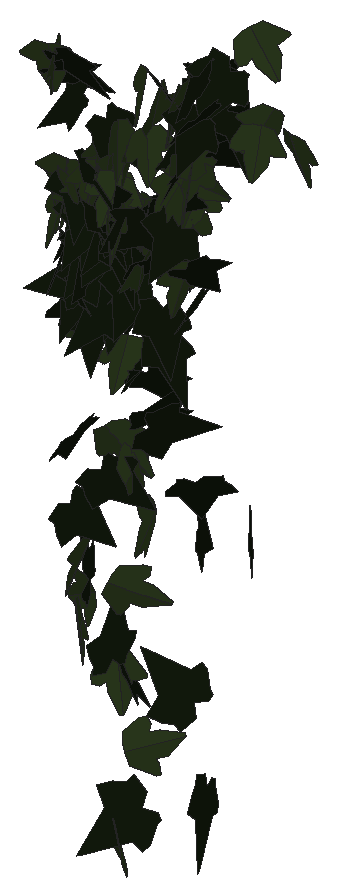
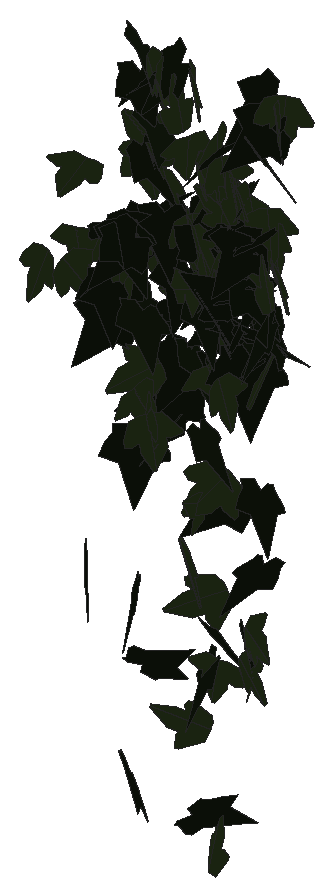
# SketchUp Ruby script. Lengths in inches.
U = 1.inch
M = Sketchup.active_model
def pt(a) = Geom::Point3d.new(a.map { |v| v * U })
def face(e, loops, mat)
  f = e.add_face(loops[0].map { |a| pt(a) })
  loops[1..].each { |l| e.add_face(l.map { |a| pt(a) }).erase! }
  f.material = f.back_material = mat if mat
  f
end
# faces: each face lists its corners as indices into pts; further lists are holes
def faces(e, pts, list, mat = nil) = list.each { |f| face(e, (f[0].is_a?(Array) ? f : [f]).map { |l| l.map { |i| pts[i] } }, mat) }
# xy, xz, yz: faces in a plane at the given z, y or x. An outline is a flat list of corners, or four numbers for a rectangle; further outlines are holes
def ring(l) = l.size == 4 ? [[l[0], l[1]], [l[2], l[1]], [l[2], l[3]], [l[0], l[3]]] : l.each_slice(2).to_a
def flat(e, list, mat, &to3) = list.each { |f| face(e, (f[0].is_a?(Array) ? f : [f]).map { |l| ring(l).map { |u, v| to3.(u, v) } }, mat) }
def xy(e, z, list, mat = nil) = flat(e, list, mat) { |x, y| [x, y, z] }
def xz(e, y, list, mat = nil) = flat(e, list, mat) { |x, z| [x, y, z] }
def yz(e, x, list, mat = nil) = flat(e, list, mat) { |y, z| [x, y, z] }
def lines(e, pts, list) = list.each { |a, b| e.add_line(pt(pts[a]), pt(pts[b])) }
# prism: a flat outline (further loops are holes) pulled along v
def prism(e, loops, v, mat = nil)
  f = face(e, loops, mat); d = Geom::Vector3d.new(v.map { |x| x * U })
  f.pushpull(f.normal.samedirection?(d) ? d.length : -d.length)
end
def box(e, o, s, mat = nil) = prism(e, [[o, [o[0] + s[0], o[1], o[2]], [o[0] + s[0], o[1] + s[1], o[2]], [o[0], o[1] + s[1], o[2]]]], [0, 0, s[2]], mat)
def at(x, y, z, deg = 0) = Geom::Transformation.translation(pt([x, y, z])) * Geom::Transformation.rotation(ORIGIN, Z_AXIS, deg.degrees)
def axes(o, x, y, z) = Geom::Transformation.new([*x, 0, *y, 0, *z, 0, *pt(o).to_a, 1])
def part(name) = M.definitions.add(name)
# library, detail: a bought-in or finely detailed component or shape, given as its bounding box
def library(name, o, s) = part(name).tap { |d| box(d.entities, o, s) }
def detail(e, o, s) = box(e.add_group.entities, o, s)
def put(e, d, t, mat = nil) = e.add_instance(d, t).tap { |i| i.material = mat if mat }
def group(e, t, mat = nil) = e.add_group.tap { |g| g.transformation = t; g.material = mat if mat }.entities
root = M.entities
M.materials.add("efeu1").color = [18, 25, 13]
M.materials.add("efeu2").color = [43, 57, 29]
c1 = part("ivyleaf_9")
p = [[1.54,2.16,1.25],[1.36,2.04,1.19],[-0.21,0.99,0.68],[-0.71,1.11,0.82],[-0.85,0.86,0.67],[-0.8,0.17,0.21],
  [-0.9,-0.01,0.1],[-0.67,-0.16,-0.02],[-0.08,-0.08,-0.05],[-0.03,-0.6,-0.4],[0.65,-0.88,-0.66],[0.83,-0.6,-0.49],
  [1.29,-0.42,-0.43],[1.8125,-0.07,-0.26],[1.21,0.44,0.15]]
faces(c1.entities,p,[[0,1,2,3,4,5,6,7,8,9,10,11,12,13,14]],"efeu1")
c2 = part("ivyleaf_10")
p = [[0,0.5,-0.03],[-0.0625,2.02,-0.43],[-0.19,2.01,-0.46],[-0.54,1.05,-0.29],[-0.52,0.625,-0.18],[-0.83,0.76,-0.28],
  [-1.16,0.64,-0.33],[-1.15,0.33,-0.24],[-0.77,-0.39,0.02],[-0.3,-0.51,0.16],[0.04,-0.48,0.23],[-0.02,2.01,-0.4375],
  [-0.06,2.01,-0.43],[0.04,-0.49,0.23],[0.67,-0.49,0.14],[1.38,0.36,-0.2],[1.375,0.51,-0.24],[0.81,0.65,-0.19],
  [0.62,0.59,-0.15],[0.6,1.09,-0.28],[0.5,1.23,-0.31]]
faces(c2.entities,p,[[0,1,2,3,4,5,6,7,8,9,10],[11,12,0,13,14,15,16,17,18,19,20]],"efeu2")
put(root,c1,axes([570.06,132.24,232.82],[0.80503,-0.25193,-0.4599],[-0.43444,0.15145,-0.84343],[0.29366,0.91468,0.01298]))
put(root,c2,axes([570.07,132.39,234.11],[0.35758,-0.85019,-0.25363],[0.0877,-0.23825,0.92226],[-0.88287,-0.36801,-0.01111]))
put(root,c1,axes([570.45,131.11,231.73],[0.17538,0.16443,1.06836],[0.09297,1.07602,-0.18087],[-1.07693,0.11967,0.15837]))
put(root,c2,axes([570.51,130.82,242.45],[-0.96058,-0.33509,0.03934],[-0.03215,-0.02726,-1.01724],[0.33585,-0.961,0.01514]))
put(root,c2,axes([570.41,131.36,234.92],[0.7141,-0.69206,-0.00415],[-0.00365,0.0022,-0.99443],[0.69207,0.71411,-0.00095]))
put(root,c2,axes([570.41,131.28,242.22],[0.48074,-0.88459,-0.03625],[0.07895,0.08391,-1.00083],[0.88181,0.47474,0.10937]))
put(root,c2,axes([570.74,131.15,236.51],[-0.90983,0.25476,0.26269],[-0.28872,-0.06724,-0.93478],[-0.22483,-0.9446,0.13739]))
put(root,c2,axes([571.03,132.55,216.36],[0.46106,-0.2348,-0.81317],[-0.63107,0.5217,-0.50845],[0.56402,0.77566,0.09583]))
put(root,c2,axes([570.85,139.36,230.89],[-0.69817,-0.66785,0.17498],[-0.06821,-0.18092,-0.96265],[0.68701,-0.69665,0.08225]))
put(root,c2,axes([570.59,132.8,218.12],[0.32909,-0.77667,0.49021],[0.17405,-0.45856,-0.84336],[0.90179,0.37193,-0.01612]))
put(root,c1,axes([571.32,132.36,217.23],[-0.49104,0.4243,-0.71417],[-0.76734,0.08611,0.57876],[0.31821,0.8624,0.29358]))
put(root,c2,axes([570.68,132.49,229.26],[-0.29802,0.71193,0.55488],[0.21221,-0.5127,0.77179],[0.87733,0.36585,0.0018]))
put(root,c1,axes([570.26,139.16,230.47],[0.36402,-0.90757,0.07302],[0.03277,-0.06553,-0.97783],[0.90991,0.36544,0.00601]))
put(root,c1,axes([571.44,131.79,231.68],[-0.80964,0.2299,0.44537],[-0.4632,-0.01997,-0.83173],[-0.19147,-0.92384,0.12881]))
put(root,c1,axes([571.05,131.61,224.2],[-0.16257,0.93149,-0.01676],[0.03186,-0.01144,-0.94512],[-0.9311,-0.16303,-0.02942]))
put(root,c2,axes([571.05,131.23,237.06],[-0.89178,-0.36298,0.18579],[-0.15683,-0.10711,-0.96202],[0.3764,-0.90461,0.03936]))
put(root,c1,axes([571.58,131.43,240.51],[-0.87516,0.48207,0.03648],[-0.03085,0.0196,-0.99914],[-0.48246,-0.8757,-0.00228]))
put(root,c1,axes([571.4,132,234.29],[-0.3315,0.76712,-0.46972],[0.06912,-0.47739,-0.82844],[-0.89684,-0.32034,0.10977]))
put(root,c1,axes([571.52,138.9,235.85],[-0.09953,0.94835,0.08723],[-0.17627,0.06785,-0.93873],[-0.9359,-0.11363,0.16752]))
put(root,c2,axes([570.63,139.5,231.6875],[0.54974,-0.43926,0.63584],[0.64486,-0.1693,-0.6745],[0.42591,0.82331,0.20054]))
put(root,c2,axes([571.24,133.97,230.12],[-0.02569,-0.94211,0.10099],[0.00022,-0.10103,-0.94246],[0.94751,-0.02552,0.00296]))
put(root,c1,axes([570.76,131.08,241.6],[0.86003,0.47043,0.25534],[0.19952,0.16666,-0.97907],[-0.49668,0.88152,0.04884]))
put(root,c1,axes([571.36,131.87,230.49],[0.4534,0.97062,-0.41574],[-0.18987,-0.37013,-1.0712],[-1.03869,0.49134,0.01433]))
put(root,c1,axes([570.94,131.71,220.78],[0.20367,-0.42553,-0.82993],[-0.16032,0.82087,-0.46023],[0.91878,0.23757,0.10367]))
put(root,c1,axes([571.66,134.79,228.26],[-0.57972,0.70231,-0.26845],[0.14614,-0.22727,-0.91015],[-0.73753,-0.59707,0.03067]))
put(root,c2,axes([571.375,139.47,232.26],[0.3097,0.78323,-0.43615],[-0.30156,-0.34354,-0.83104],[-0.84424,0.41003,0.13685]))
put(root,c2,axes([571.46,131.82,235.83],[-0.32952,-0.86435,0.28217],[-0.03389,-0.28825,-0.92253],[0.90861,-0.32421,0.06793]))
put(root,c1,axes([571.18,131.99,236.23],[-0.17021,-0.95833,0.01524],[0.01859,-0.01877,-0.97309],[0.95827,-0.16985,0.02159]))
put(root,c1,axes([571.5,131.72,231.66],[-0.80182,-0.36143,-0.36519],[0.3775,0.04477,-0.87315],[0.34855,-0.87993,0.10558]))
put(root,c1,axes([571.44,131.9,236.125],[0.53595,0.77957,0.25222],[0.14579,0.20585,-0.94602],[-0.80628,0.55541,-0.00339]))
put(root,c1,axes([571.24,130.55,242.59],[0.993,0.18995,0.03398],[0.03615,-0.00816,-1.0109],[-0.18955,0.99355,-0.0148]))
put(root,c1,axes([571.47,132.28,229.91],[-0.03325,-0.9598,-0.02296],[-0.01292,0.02342,-0.96028],[0.95999,-0.03293,-0.01372]))
put(root,c2,axes([571.39,131.58,215.92],[-0.33428,0.62383,-0.84867],[0.39543,-0.75093,-0.70773],[-0.97624,-0.51778,0.00393]))
put(root,c1,axes([571.3,131.54,231.25],[0.77282,-0.60709,0.0565],[0.04099,-0.03928,-0.98274],[0.60834,0.77389,-0.00556]))
put(root,c1,axes([572,131.83,235.03],[-0.74465,-0.60263,-0.04579],[0.04449,0.0178,-0.95784],[0.60272,-0.74585,0.01413]))
put(root,c2,axes([571.37,138.6875,233.17],[0.48259,0.11114,0.84976],[0.48705,0.76686,-0.37689],[-0.70515,0.60573,0.32124]))
put(root,c1,axes([572.02,132.18,233.34],[-0.57787,-0.7499,0.17358],[-0.10287,-0.13987,-0.94671],[0.76282,-0.58694,0.00383]))
put(root,c1,axes([571.59,132.27,232.28],[0.27664,-0.27868,-0.87738],[0.62504,-0.61575,0.39266],[-0.67587,-0.68351,0.004]))
put(root,c2,axes([572.3125,131.54,237.27],[-0.2833,-0.90798,0.17177],[0.0667,-0.19929,-0.94341],[0.92168,-0.26467,0.12107]))
put(root,c1,axes([572.08,132.1,236.54],[-0.47191,-0.66497,-0.52291],[0.30279,0.42633,-0.81541],[0.7899,-0.5607,0.00016]))
put(root,c2,axes([572.76,137.95,236.44],[-0.30967,0.6152,0.70883],[-0.49007,0.5306,-0.67461],[-0.80047,-0.56285,0.1388]))
put(root,c2,axes([572.45,131.34,237.875],[0.65649,-0.72856,0.031],[0.04525,-0.00094,-0.98015],[0.72782,0.65722,0.03297]))
put(root,c1,axes([572.91,138.375,238.94],[-0.16515,0.90966,-0.30338],[-0.0851,-0.32053,-0.91477],[-0.95513,-0.12873,0.13396]))
put(root,c2,axes([572.33,131.79,237.34],[0.37838,-0.88399,-0.20248],[0.06558,-0.19215,0.96145],[-0.90451,-0.38373,-0.015]))
put(root,c1,axes([572.16,132.23,233.17],[-0.12118,-0.04696,0.95522],[0.90753,0.29812,0.12979],[-0.30172,0.91556,0.00673]))
put(root,c1,axes([572.15,131.46,237.55],[0.57878,-0.79009,-0.00887],[0.00347,0.01353,-0.97934],[0.79013,0.57869,0.01079]))
put(root,c1,axes([572.36,138.53,238.96],[0.90513,0.36895,0.04233],[0.03833,0.01809,-0.97743],[-0.36939,0.90594,0.00228]))
put(root,c1,axes([572.26,131.79,235.17],[0.50367,-0.8208,-0.00799],[0.0468,0.03807,-0.96116],[0.81951,0.50229,0.0598]))
put(root,c2,axes([572.47,131.73,237.125],[-0.4335,-0.53228,0.70794],[0.44133,0.55357,0.68646],[-0.76795,0.6186,-0.00514]))
put(root,c1,axes([573.25,131.16,231.32],[-0.98427,-0.05458,-0.09049],[0.09,0.01136,-0.98577],[0.05538,-0.98836,-0.00633]))
put(root,c1,axes([573.1,138.91,236.83],[0.31007,0.86617,-0.28105],[-0.13665,-0.24928,-0.91901],[-0.90032,0.33614,0.04269]))
put(root,c2,axes([573.11,131.55,238.95],[-0.24491,-0.9614,-0.02234],[-0.00535,0.02441,-0.99204],[0.96164,-0.24471,-0.0112]))
put(root,c2,axes([573.17,138.45,238.46],[-0.72614,-0.64271,0.01976],[-0.01782,-0.00969,-0.96971],[0.64277,-0.72634,-0.00455]))
put(root,c1,axes([573.68,132.07,232.42],[-0.38396,0.56598,0.6905],[-0.39616,0.5656,-0.68389],[-0.80012,-0.55165,0.00726]))
put(root,c2,axes([572.71,132.32,224.52],[-0.92825,-0.10382,-0.68038],[0.6769,0.06889,-0.93403],[0.12447,-1.14883,0.00548]))
put(root,c1,axes([573.4,131.67,235.11],[-0.94364,-0.06464,-0.21251],[0.21457,-0.02559,-0.94503],[0.0574,-0.96693,0.03922]))
put(root,c2,axes([572.68,132.18,231.24],[0.6016,-0.3423,0.67466],[0.58303,-0.33951,-0.69215],[0.48209,0.83775,-0.00484]))
put(root,c1,axes([573.09,132.22,231.59],[-0.37575,-0.88439,-0.09622],[0.02409,0.0943,-0.96079],[0.88928,-0.37624,-0.01463]))
put(root,c2,axes([573.09,131.73,235.16],[-0.17439,0.78244,-0.53018],[0.10337,-0.52011,-0.80157],[-0.93948,-0.20247,0.01022]))
put(root,c1,axes([572.85,131.39,223.22],[-0.01193,-0.22479,-0.93849],[0.23992,0.90841,-0.22063],[0.93474,-0.23603,0.04465]))
put(root,c1,axes([573.11,138.71,235.2],[0.6846,0.68212,0.23219],[0.15541,0.17296,-0.96634],[-0.7036,0.70191,0.01248]))
put(root,c1,axes([573.75,132.04,232.42],[-0.24131,0.93783,0.0854],[-0.01278,0.08489,-0.96834],[-0.94162,-0.24149,-0.00875]))
put(root,c1,axes([572.96,132.11,233.6],[0.36008,-0.89443,0.10005],[0.04822,-0.08844,-0.96412],[0.89871,0.36311,0.01164]))
put(root,c2,axes([573.54,132,234.63],[0.09297,-0.93451,0.23239],[-0.0068,-0.2341,-0.93867],[0.96294,0.08857,-0.02907]))
put(root,c2,axes([573.47,131.34,236.97],[0.8917,0.3146,-0.20741],[-0.1995,-0.05787,-0.9455],[-0.31967,0.91367,0.01153]))
put(root,c2,axes([574.08,132.34,235.65],[-0.7996,-0.00173,0.54563],[-0.53066,-0.22275,-0.77836],[0.12694,-0.94205,0.18304]))
put(root,c2,axes([573.62,132.07,223.05],[0.0878,0.40548,-0.90284],[0.10019,0.89809,0.41309],[0.98464,-0.12754,0.03847]))
put(root,c1,axes([573.68,132.19,232.28],[-0.81495,-0.45221,-0.25531],[0.28306,0.01149,-0.92389],[0.43537,-0.85393,0.12277]))
put(root,c1,axes([573.16,131.3,239.88],[0.51193,-0.72194,-0.47513],[-0.03785,0.53297,-0.85061],[0.86343,0.4514,0.24442]))
put(root,c1,axes([573.75,138.42,239.21],[-0.60571,-0.75027,0.13069],[-0.1021,-0.08547,-0.96392],[0.7547,-0.61373,-0.02552]))
put(root,c2,axes([573.65,131.77,229.18],[0.48466,0.78049,-0.29783],[-0.16497,-0.24813,-0.91868],[-0.81893,0.51189,0.0088]))
put(root,c1,axes([574.08,130.41,215.36],[-0.92822,0.41046,-0.14762],[-0.14699,0.03244,1.0145],[0.41068,0.93933,0.02947]))
put(root,c1,axes([573.82,132.01,235.03],[0.51456,0.37373,0.736],[-0.58363,-0.44861,0.63582],[0.58374,-0.77796,-0.01307]))
put(root,c2,axes([573.67,131.13,235.86],[0.85576,-0.40605,0.19881],[0.19672,-0.04877,-0.94639],[0.40707,0.87719,0.03942]))
put(root,c2,axes([573.93,131.16,205.52],[-0.8462,0.58583,0.16938],[0.13526,-0.10219,1.02918],[0.59463,0.85692,0.00694]))
put(root,c1,axes([573.49,139.1875,236.92],[0.1829,-0.94512,-0.01882],[0.07328,0.03329,-0.95947],[0.94246,0.18083,0.07826]))
put(root,c2,axes([574.11,132.79,220.83],[0.75436,-0.82872,-0.33081],[-0.22945,0.23847,-1.1206],[0.8623,0.78843,-0.00878]))
put(root,c2,axes([573.9375,131.9375,238.78],[0.4551,-0.80039,0.327],[0.1639,-0.28297,-0.92073],[0.84894,0.48371,0.00246]))
put(root,c2,axes([573.99,130.95,239.78],[-0.13703,0.94177,-0.27405],[-0.05291,-0.28341,-0.94747],[-0.97941,-0.11646,0.08953]))
put(root,c1,axes([574.4375,131.72,207.68],[-0.72498,-0.66511,0.54562],[-0.38692,-0.38518,-0.98366],[0.76835,-0.82154,0.01947]))
put(root,c1,axes([573.95,131.99,232.125],[-0.21991,-0.8844,0.3419],[-0.00764,-0.34931,-0.90849],[0.94816,-0.20794,0.07197]))
put(root,c1,axes([574.09,131.07,214.74],[0.75155,-0.19926,-0.68491],[-0.63154,0.27667,-0.77347],[0.33162,0.97847,0.07922]))
put(root,c2,axes([573.86,130.93,214.64],[0.95656,0.23973,0.27],[0.2586,0.07869,-0.98606],[-0.25198,0.99082,0.01298]))
put(root,c2,axes([574.32,131.97,233.125],[0.11153,-0.95978,-0.13196],[-0.00346,0.13244,-0.96617],[0.9688,0.11096,0.01175]))
put(root,c2,axes([574.43,131.93,235.95],[-0.55119,-0.8014,0.07954],[0.05117,-0.13104,-0.96571],[0.80371,-0.54126,0.11603]))
put(root,c2,axes([573.79,133.07,233.65],[-0.42089,0.02648,-0.86094],[0.79149,-0.36613,-0.3982],[-0.3398,-0.88562,0.13888]))
put(root,c2,axes([573.84,131.28,218.24],[-0.41731,-0.16365,-0.98224],[0.90396,0.38442,-0.4481],[0.41765,-0.99557,-0.01157]))
put(root,c1,axes([574.76,131.91,233.64],[0.25935,0.94034,0.06226],[0.01405,0.06071,-0.97544],[-0.94229,0.25971,0.00259]))
put(root,c2,axes([574.52,131.98,235.98],[0.69765,-0.67705,0.08199],[0.13525,0.02239,-0.96594],[0.66845,0.7021,0.10986]))
put(root,c1,axes([575.17,131.05,229.25],[-0.46901,0.83705,0.12655],[-0.07185,0.10479,-0.95943],[-0.84351,-0.47435,0.01136]))
put(root,c1,axes([575.23,131.07,235.9],[0.08194,0.35207,-0.91618],[-0.53512,-0.75468,-0.33787],[-0.82279,0.52589,0.1285]))
put(root,c2,axes([575,139.44,237.11],[-0.29281,-0.72583,0.57557],[-0.07949,-0.58172,-0.77403],[0.92293,-0.28038,0.11594]))
put(root,c1,axes([575.1,134.88,219.78],[0.28624,-0.09926,-0.94411],[-0.83979,0.43334,-0.30017],[0.44266,0.88628,0.04103]))
put(root,c2,axes([575,131.22,242.46],[0.6797,-0.73774,0.09596],[0.12588,-0.01406,-0.99971],[0.73323,0.6863,0.08267]))
put(root,c2,axes([574.97,131.58,239.55],[0.36268,0.90878,-0.04945],[-0.02709,-0.04243,-0.97843],[-0.90972,0.36357,0.00943]))
put(root,c1,axes([575.44,132.53,236.33],[0.2755,0.85003,-0.3728],[-0.16556,-0.33764,-0.8922],[-0.91331,0.31761,0.04928]))
put(root,c2,axes([575.31,131.71,240.61],[0.13341,-0.96725,-0.13885],[0.01698,-0.13782,0.97641],[-0.97702,-0.13448,-0.00199]))
put(root,c1,axes([575.54,130.99,228.94],[0.75406,0.60791,-0.08571],[-0.05848,-0.06402,-0.9685],[-0.61113,0.75621,-0.01308]))
put(root,c1,axes([575.23,131.5,226.34],[0.6624,0.73295,0.16831],[-0.11536,-0.1226,0.98792],[0.74313,-0.67236,0.00334]))
put(root,c2,axes([575.24,138.34,241.4375],[0.63917,0.58498,0.50192],[0.39359,0.31292,-0.86593],[-0.66273,0.75003,-0.03019]))
put(root,c2,axes([575.14,130.72,211.29],[0.34309,0.03843,-0.97279],[0.93722,0.26609,0.34106],[0.26346,-0.9966,0.05355]))
put(root,c2,axes([576.24,131.59,237.48],[0.84611,-0.36772,-0.35356],[-0.31061,0.17182,-0.92202],[0.40465,0.90077,0.03155]))
put(root,c2,axes([576.04,137.54,237.4],[0.94703,0.25315,-0.02818],[-0.03878,0.03606,-0.97926],[-0.25175,0.94676,0.04483]))
put(root,c1,axes([575.87,131.5,231.75],[0.037,-0.95839,-0.1884],[-0.02595,0.1875,-0.95892],[0.97638,0.0413,-0.01835]))
put(root,c1,axes([575.81,131.11,242.82],[0.94921,-0.21762,-0.23757],[-0.22719,0.07196,-0.97366],[0.22844,0.97584,0.01882]))
put(root,c1,axes([576.78,131.29,239.68],[-0.01523,0.80097,0.56558],[-0.26396,0.54141,-0.77386],[-0.94432,-0.16426,0.20719]))
put(root,c1,axes([576.8,132.2,238.93],[-0.47876,0.73254,-0.44404],[0.19211,-0.40391,-0.87347],[-0.83479,-0.51307,0.05365]))
put(root,c1,axes([577.25,131.62,213.85],[-0.85661,-0.51484,-0.34167],[-0.29441,-0.1734,0.99942],[-0.54325,0.90579,-0.00287]))
put(root,c1,axes([576.09,131.35,230.55],[0.26091,-0.95777,-0.20472],[0.0261,0.21859,-0.98937],[0.97906,0.24941,0.08093]))
put(root,c1,axes([576.8,131.85,231.63],[0.17866,0.59175,0.76323],[-0.06452,0.78176,-0.59101],[-0.9636,0.05737,0.18109]))
put(root,c2,axes([576.86,132.13,238.58],[-0.81688,-0.46461,0.26942],[-0.17083,-0.24017,-0.93213],[0.50918,-0.82595,0.1195]))
put(root,c1,axes([576.22,130.375,226.9],[0.10236,0.39849,-0.95616],[0.05916,0.957,0.40517],[1.03419,-0.09418,0.07146]))
put(root,c1,axes([576.6,131.67,235.79],[-0.40733,-0.82366,0.36064],[-0.01719,-0.38872,-0.9072],[0.89899,-0.38063,0.14606]))
put(root,c2,axes([576.4,131.64,241.91],[0.50796,-0.56051,0.63878],[0.42809,-0.4741,-0.75643],[0.73413,0.66429,-0.00088]))
put(root,c2,axes([576.76,139.12,236.66],[-0.92267,0.37899,-0.11821],[0.11416,-0.03317,-0.99739],[-0.38023,-0.92962,-0.01261]))
put(root,c2,axes([576.9,131.56,242.5625],[0.38981,-0.90322,0.13286],[0.06076,-0.11848,-0.98371],[0.91092,0.39442,0.00876]))
put(root,c2,axes([577.04,131.5,234.03],[-0.14214,-0.9101,0.34763],[0.10118,-0.3632,-0.90949],[0.96896,-0.09559,0.14596]))
put(root,c2,axes([577.05,131.63,238.88],[-0.18492,-0.85888,0.45642],[0.08703,0.44813,0.87852],[-0.96872,0.20421,-0.0082]))
put(root,c2,axes([577.08,131.61,238.57],[0.67501,-0.67362,0.27035],[0.24447,-0.13663,-0.95082],[0.68343,0.71418,0.0731]))
put(root,c1,axes([577.72,134.98,220.38],[0.18354,-0.04758,-0.98882],[-0.95506,0.25616,-0.1896],[0.26054,0.97254,0.00156]))
put(root,c1,axes([577.2,132.67,209.11],[-0.67999,0.04374,-0.95208],[0.94696,-0.10136,-0.68099],[-0.10787,-1.16558,0.02349]))
put(root,c1,axes([578.02,130.8125,242.83],[-0.236,0.73124,0.63325],[-0.26807,0.57686,-0.76603],[-0.92944,-0.35206,0.06014]))
put(root,c1,axes([577.85,131.16,241.64],[-0.19566,0.96299,-0.1223],[0.01578,-0.12158,-0.98263],[-0.9706,-0.1961,0.00867]))
put(root,c1,axes([577.51,131.09,234.52],[0.5824,0.79379,0.0726],[0.03373,0.06528,-0.98447],[-0.79639,0.58327,0.01139]))
put(root,c1,axes([577.74,131.38,224.33],[0.47522,0.81082,-0.33488],[-0.2131,-0.26276,-0.93859],[-0.85098,0.51859,0.04803]))
put(root,c1,axes([577.6,131.59,241.3125],[-0.22435,-0.88497,0.38336],[0.01131,-0.39598,-0.90749],[0.96437,-0.20123,0.09983]))
